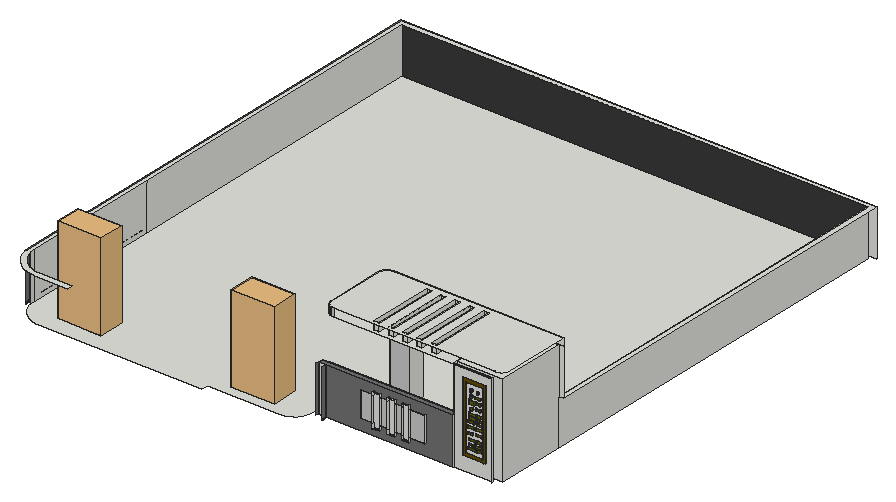
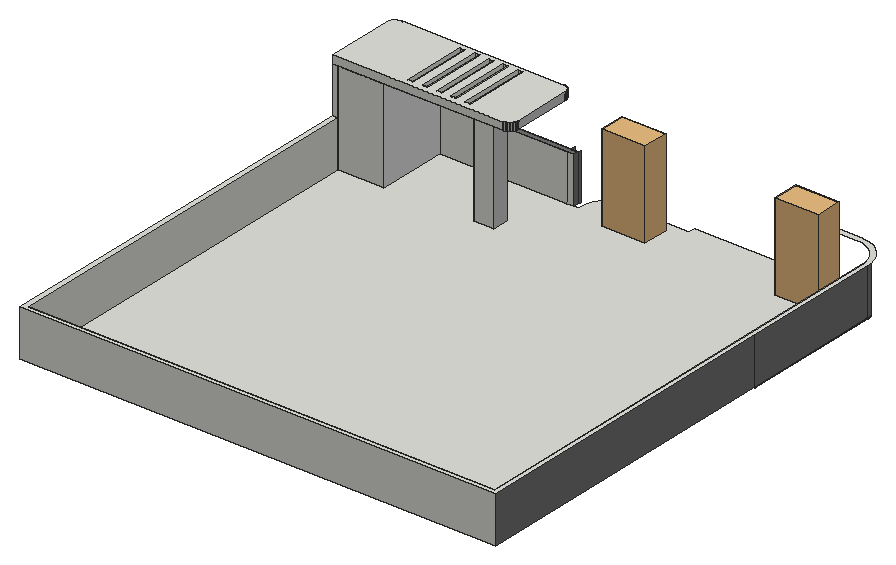
# SketchUp Ruby script. Lengths in inches.
U = 1.inch
M = Sketchup.active_model
def pt(a) = Geom::Point3d.new(a.map { |v| v * U })
def face(e, loops, mat)
  f = e.add_face(loops[0].map { |a| pt(a) })
  loops[1..].each { |l| e.add_face(l.map { |a| pt(a) }).erase! }
  f.material = f.back_material = mat if mat
  f
end
# faces: each face lists its corners as indices into pts; further lists are holes
def faces(e, pts, list, mat = nil) = list.each { |f| face(e, (f[0].is_a?(Array) ? f : [f]).map { |l| l.map { |i| pts[i] } }, mat) }
# xy, xz, yz: faces in a plane at the given z, y or x. An outline is a flat list of corners, or four numbers for a rectangle; further outlines are holes
def ring(l) = l.size == 4 ? [[l[0], l[1]], [l[2], l[1]], [l[2], l[3]], [l[0], l[3]]] : l.each_slice(2).to_a
def flat(e, list, mat, &to3) = list.each { |f| face(e, (f[0].is_a?(Array) ? f : [f]).map { |l| ring(l).map { |u, v| to3.(u, v) } }, mat) }
def xy(e, z, list, mat = nil) = flat(e, list, mat) { |x, y| [x, y, z] }
def xz(e, y, list, mat = nil) = flat(e, list, mat) { |x, z| [x, y, z] }
def yz(e, x, list, mat = nil) = flat(e, list, mat) { |y, z| [x, y, z] }
def lines(e, pts, list) = list.each { |a, b| e.add_line(pt(pts[a]), pt(pts[b])) }
# prism: a flat outline (further loops are holes) pulled along v
def prism(e, loops, v, mat = nil)
  f = face(e, loops, mat); d = Geom::Vector3d.new(v.map { |x| x * U })
  f.pushpull(f.normal.samedirection?(d) ? d.length : -d.length)
end
def box(e, o, s, mat = nil) = prism(e, [[o, [o[0] + s[0], o[1], o[2]], [o[0] + s[0], o[1] + s[1], o[2]], [o[0], o[1] + s[1], o[2]]]], [0, 0, s[2]], mat)
def at(x, y, z, deg = 0) = Geom::Transformation.translation(pt([x, y, z])) * Geom::Transformation.rotation(ORIGIN, Z_AXIS, deg.degrees)
def axes(o, x, y, z) = Geom::Transformation.new([*x, 0, *y, 0, *z, 0, *pt(o).to_a, 1])
def part(name) = M.definitions.add(name)
# library, detail: a bought-in or finely detailed component or shape, given as its bounding box
def library(name, o, s) = part(name).tap { |d| box(d.entities, o, s) }
def detail(e, o, s) = box(e.add_group.entities, o, s)
def put(e, d, t, mat = nil) = e.add_instance(d, t).tap { |i| i.material = mat if mat }
def group(e, t, mat = nil) = e.add_group.tap { |g| g.transformation = t; g.material = mat if mat }.entities
root = M.entities
M.materials.add("[Cladding Stucco White]").color = [200, 200, 200]
M.materials.add("[Color D08]").color = [102, 76, 0]
M.materials.add("[Color E08]").color = [102, 102, 0]
M.materials.add("[Color M01]").color = [226, 226, 226]
M.materials.add("[Color M05]").color = [114, 114, 114]
M.materials.add("[Color M07]").color = [58, 58, 58]
c1 = library("Plant 260 020",[-18.86,-7.03,0.01],[33.61,20.04,67.26])
xy(root,252,[[[24.37,4.65,150.375,4.65,150.375,10.04,205.76,10.04,207.83,10.17,209.75,10.55,211.6,11.18,213.35,12.05,214.98,13.13,216.45,14.42,217.74,15.9,218.83,17.52,219.69,19.28,220.32,21.13,220.7,23.05,221.07,28.65,328.65,28.65,328.65,82.27,364.23,82.27,364.23,381.35,3.9,381.35,3.9,25.12,4.08,22.34,4.6,19.73,5.45,17.21,6.63,14.83,8.11,12.61,9.86,10.61,11.86,8.86,14.08,7.38,16.46,6.2,18.98,5.35,21.59,4.83],[244.86,68.42,260.42,80.36]],[229.875,24.5625,328.65,25]])
xy(root,257.79,[[267.39,23,273.02,24.5625],[279.08,23,284.71,24.5625],[290.02,23,295.64,24.5625]])
xy(root,261.06,[[257.61,24,267.39,24.5625],[273.02,24,279.08,24.5625],[284.71,24,290.02,24.5625],[295.64,24,307.42,24.5625]])
xy(root,262.61,[[336.12,24.6,353.93,25]])
xy(root,264.9375,[[338.45,24.6,351.61,25]],"[Color D08]")
xy(root,268.33,[[340.3,24.6,345.92,25]])
xy(root,268.45,[[347.23,24.6,350.79,25]])
xy(root,269.83,[[340.3,24.6,345.92,25]],"[Color E08]")
xy(root,270.39,[[347.23,24.6,350.79,25]],"[Color E08]")
xy(root,271.27,[[345.53,24.6,351.15,25]])
xy(root,271.58,[[340.9375,24.6,344.6875,25]])
xy(root,272.77,[[345.53,24.6,351.15,25]],"[Color E08]")
xy(root,272.83,[[340.9375,24.6,344.6875,25]],"[Color E08]")
xy(root,274.45,[[347.23,24.6,350.79,25]])
xy(root,274.58,[[340.52,24.6,346.15,25]])
xy(root,276.08,[[340.52,24.6,346.15,25]],"[Color E08]")
xy(root,276.39,[[347.23,24.6,350.79,25]],"[Color E08]")
xy(root,279.15,[[340.1875,24.6,343.9375,25]])
xy(root,279.31,[[346.11,24.6,351.49,25]])
xy(root,280.31,[[257.61,24,267.39,24.5625],[273.02,24,279.08,24.5625],[284.71,24,290.02,24.5625],[295.64,24,307.42,24.5625]])
xy(root,280.4,[[340.1875,24.6,343.9375,25]],"[Color E08]")
xy(root,280.87,[[346.11,24.6,351.49,25]],"[Color E08]")
xy(root,283.04,[[267.39,23,273.02,24.5625],[290.02,23,295.64,24.5625]])
xy(root,283.04,[[279.08,23,284.71,24.5625]],"[Color M01]")
xy(root,283.31,[[340.11,24.6,345.49,25],[346.11,24.6,351.49,25]])
xy(root,284.87,[[340.11,24.6,345.49,25],[346.11,24.6,351.49,25]],"[Color E08]")
xy(root,286.82,[[347.26,24.6,351.01,25]])
xy(root,286.87,[[340.11,24.6,345.49,25]])
xy(root,288,[[24.25,1,49.81,1,49.81,4.65,24.37,4.65,21.59,4.83,18.98,5.35,16.46,6.2,14.08,7.38,11.86,8.86,9.86,10.61,8.11,12.61,6.63,14.83,5.45,17.21,4.6,19.73,4.08,22.34,3.9,25.12,3.9,381.35,364.23,381.35,364.23,82.27,367.875,82.27,367.875,385,0.25,385,0.25,25,0.46,21.87,1.07,18.79,2.08,15.82,3.47,13,5.21,10.39,7.28,8.03,9.64,5.96,12.25,4.22,15.07,2.83,18.04,1.82,21.12,1.21]])
xy(root,288,[[229.875,24.5625,328.65,24.5625,328.65,28.65,224.48,28.65,224.48,25,229.875,25]],"[Color M05]")
xy(root,288.07,[[347.26,24.6,351.01,25]],"[Color E08]")
xy(root,288.43,[[340.11,24.6,345.49,25]],"[Color E08]")
xy(root,289.68,[[340.68,24.6,346.49,25]])
xy(root,289.75,[[347.26,24.6,351.01,25]])
xy(root,291,[[347.26,24.6,351.01,25]],"[Color E08]")
xy(root,291.43,[[340.68,24.6,346.49,25]],"[Color E08]")
xy(root,292.39,[[340.52,24.6,346.15,25]])
xy(root,292.44,[[346.69,24.6,350.25,25]])
xy(root,293.89,[[340.52,24.6,346.15,25]],"[Color E08]")
xy(root,294.38,[[346.69,24.6,350.25,25]],"[Color E08]")
xy(root,296.78,[[346.22,24.6,350.21,25]])
xy(root,298.625,[[346.22,24.6,350.21,25]],"[Color E08]")
xy(root,300.12,[[340.54,24.6,344.89,25]])
xy(root,300.97,[[345.92,24.6,349.92,25]])
xy(root,302.59,[[345.92,24.6,349.92,25]],"[Color E08]")
xy(root,302.8,[[340.54,24.6,344.89,25]],"[Color E08]")
xy(root,305.05,[[345.58,24.6,350.08,25]])
xy(root,306.3,[[345.58,24.6,350.08,25]],"[Color E08]")
xy(root,314.59,[[338.45,24.6,351.61,25]])
xy(root,316.92,[[336.12,24.6,353.93,25]],"[Color D08]")
xy(root,324,[[[236.52,24,235.66,24.06,234.8,24.23,233.98,24.51,233.2,24.89,232.48,25.375,231.82,25.95,231.25,26.6,230.77,27.32,230.38,28.1,230.1,28.93,229.93,29.78,229.875,30.65,229.875,75.46,229.93,76.35,230.11,77.22,230.39,78.07,230.79,78.86,231.28,79.61,231.87,80.28,232.54,80.86,233.28,81.36,234.08,81.75,234.92,82.04,235.8,82.21,236.6875,82.27,328.65,82.27,328.65,25,358.875,25,358.875,24],[265.73,27.1,269.54,77.6],[276.79,27.1,280.6,77.6],[287.85,27.1,291.66,77.6],[298.91,27.1,302.73,77.6],[309.98,27.1,313.79,77.6],[244.86,68.42,260.42,80.36]],[328.65,28.65,364.23,82.27]])
xy(root,330,[[361.5,23.99,361.5625,24,360.74,24],[[236.52,24,361.5625,24,362.25,24.07,362.99,24.22,363.72,24.45,364.41,24.76,365.07,25.14,365.68,25.58,366.24,26.09,366.75,26.65,367.19,27.27,367.57,27.92,367.875,28.62,367.875,82.27,236.6875,82.27,235.8,82.21,234.92,82.04,234.08,81.75,233.28,81.36,232.54,80.86,231.87,80.28,231.28,79.61,230.79,78.86,230.39,78.07,230.11,77.22,229.93,76.35,229.875,75.46,229.875,30.65,229.93,29.78,230.1,28.93,230.38,28.1,230.77,27.32,231.25,26.6,231.82,25.95,232.48,25.375,233.2,24.89,233.98,24.51,234.8,24.23,235.66,24.06],[265.73,27.1,269.54,77.6],[276.79,27.1,280.6,77.6],[287.85,27.1,291.66,77.6],[309.98,27.1,313.79,77.6],[298.91,27.1,302.73,77.6]]])
xz(root,24,[[257.61,261.06,267.39,280.31],[273.02,261.06,279.08,280.31],[284.71,261.06,290.02,280.31],[295.64,261.06,307.42,280.31]],"[Cladding Stucco White]")
xz(root,24.5625,[[[229.875,252,328.65,288],[267.39,257.79,267.39,261.06,257.61,261.06,257.61,280.31,267.39,280.31,267.39,283.04,273.02,283.04,273.02,280.31,279.08,280.31,279.08,283.04,284.71,283.04,284.71,280.31,290.02,280.31,290.02,283.04,295.64,283.04,295.64,280.31,307.42,280.31,307.42,261.06,295.64,261.06,295.64,257.79,290.02,257.79,290.02,261.06,284.71,261.06,284.71,257.79,279.08,257.79,279.08,261.06,273.02,261.06,273.02,257.79]]],"[Color M05]")
xz(root,24.6,[[[336.12,262.61,353.93,316.92],[338.45,264.9375,351.61,314.59]]],"[Color D08]")
xz(root,24.6,[[340.3,268.33,345.92,269.83],[347.23,268.45,350.79,270.39],[345.53,271.27,351.15,272.77],[340.9375,271.58,344.6875,272.83],[347.23,274.45,350.79,276.39],
  [340.52,274.58,346.15,276.08],[340.1875,279.15,343.9375,280.4],[346.11,279.31,351.49,280.87],[340.11,283.31,345.49,284.87],[346.11,283.31,351.49,284.87],
  [347.26,286.82,351.01,288.07],[340.11,286.87,345.49,288.43],[340.68,289.68,346.49,291.43],[347.26,289.75,351.01,291],[340.52,292.39,346.15,293.89],
  [346.69,292.44,350.25,294.38],[343.01,295.6,343.3125,295.64,343.6,295.76,343.85,295.94,344.03,296.19,344.15,296.48,344.19,296.78,344.15,297.09,344.03,297.38,343.85,297.625,343.6,297.8125,343.3125,297.93,343.01,297.97,342.7,297.93,342.41,297.8125,342.17,297.625,341.98,297.38,341.86,297.09,341.82,296.78,341.86,296.48,341.98,296.19,342.17,295.94,342.41,295.76,342.7,295.64],[346.22,296.78,350.21,298.625],[340.54,300.12,344.89,302.8],[345.92,300.97,349.92,302.59],
  [342.68,304.3125,342.98,304.35,343.25,304.46,343.48,304.64,343.66,304.875,343.77,305.15,343.81,305.4375,343.77,305.73,343.66,306,343.48,306.23,343.25,306.41,342.98,306.52,342.68,306.5625,342.39,306.52,342.12,306.41,341.89,306.23,341.71,306,341.6,305.73,341.56,305.4375,341.6,305.15,341.71,304.875,341.89,304.64,342.12,304.46,342.39,304.35],[345.58,305.05,350.08,306.3],[342.68,308.51,342.99,308.55,343.28,308.67,343.52,308.86,343.71,309.11,343.83,309.39,343.87,309.7,343.83,310.01,343.71,310.3,343.52,310.54,343.28,310.73,342.99,310.85,342.68,310.89,342.375,310.85,342.09,310.73,341.84,310.54,341.66,310.3,341.54,310.01,341.5,309.7,341.54,309.39,341.66,309.11,341.84,308.86,342.09,308.67,342.375,308.55],[347.69,308.5625,347.93,308.6,348.16,308.6875,348.35,308.84,348.5,309.03,348.6,309.26,348.63,309.5,348.6,309.74,348.5,309.97,348.35,310.16,348.16,310.3125,347.93,310.41,347.69,310.4375,347.45,310.41,347.22,310.3125,347.03,310.16,346.88,309.97,346.79,309.74,346.75,309.5,346.79,309.26,346.88,309.03,347.03,308.84,347.22,308.6875,347.45,308.6]],"[Color E08]")
xz(root,25,[[224.48,252,229.875,288],[[328.65,252,358.875,324],[336.12,262.61,353.93,316.92]]])
xz(root,25,[[[338.45,264.9375,351.61,314.59],[340.54,300.12,344.89,302.8],[340.68,289.68,346.49,291.43],[340.52,292.39,346.15,293.89],[340.52,274.58,346.15,276.08],[345.53,271.27,351.15,272.77],[340.3,268.33,345.92,269.83],[340.11,286.87,345.49,288.43],[340.11,283.31,345.49,284.87],[346.11,283.31,351.49,284.87],[346.11,279.31,351.49,280.87],[346.22,296.78,350.21,298.625],[346.69,292.44,350.25,294.38],[347.23,274.45,350.79,276.39],[347.23,268.45,350.79,270.39],[345.92,300.97,349.92,302.59],[345.58,305.05,350.08,306.3],[347.26,289.75,351.01,291],[347.26,286.82,351.01,288.07],[340.1875,279.15,343.9375,280.4],[340.9375,271.58,344.6875,272.83],[342.68,308.51,342.375,308.55,342.09,308.67,341.84,308.86,341.66,309.11,341.54,309.39,341.5,309.7,341.54,310.01,341.66,310.3,341.84,310.54,342.09,310.73,342.375,310.85,342.68,310.89,342.99,310.85,343.28,310.73,343.52,310.54,343.71,310.3,343.83,310.01,343.87,309.7,343.83,309.39,343.71,309.11,343.52,308.86,343.28,308.67,342.99,308.55],[343.01,295.6,342.7,295.64,342.41,295.76,342.17,295.94,341.98,296.19,341.86,296.48,341.82,296.78,341.86,297.09,341.98,297.38,342.17,297.625,342.41,297.8125,342.7,297.93,343.01,297.97,343.3125,297.93,343.6,297.8125,343.85,297.625,344.03,297.38,344.15,297.09,344.19,296.78,344.15,296.48,344.03,296.19,343.85,295.94,343.6,295.76,343.3125,295.64],[342.68,304.3125,342.39,304.35,342.12,304.46,341.89,304.64,341.71,304.875,341.6,305.15,341.56,305.4375,341.6,305.73,341.71,306,341.89,306.23,342.12,306.41,342.39,306.52,342.68,306.5625,342.98,306.52,343.25,306.41,343.48,306.23,343.66,306,343.77,305.73,343.81,305.4375,343.77,305.15,343.66,304.875,343.48,304.64,343.25,304.46,342.98,304.35],[347.69,308.5625,347.45,308.6,347.22,308.6875,347.03,308.84,346.88,309.03,346.79,309.26,346.75,309.5,346.79,309.74,346.88,309.97,347.03,310.16,347.22,310.3125,347.45,310.41,347.69,310.4375,347.93,310.41,348.16,310.3125,348.35,310.16,348.5,309.97,348.6,309.74,348.63,309.5,348.6,309.26,348.5,309.03,348.35,308.84,348.16,308.6875,347.93,308.6]]],"[Color M01]")
xz(root,27.1,[[265.73,324,269.54,330],[276.79,324,280.6,330],[287.85,324,291.66,330],[298.91,324,302.73,330],[309.98,324,313.79,330]])
xz(root,28.65,[[224.48,252,229.875,288],[229.875,252,328.65,288],[328.65,252,364.23,324]])
xz(root,68.42,[[244.86,252,260.42,324]],"[Cladding Stucco White]")
xz(root,77.6,[[265.73,324,269.54,330],[276.79,324,280.6,330],[287.85,324,291.66,330],[298.91,324,302.73,330],[309.98,324,313.79,330]])
xz(root,80.36,[[244.86,252,260.42,324]])
xz(root,82.27,[[328.65,252,364.23,324],[364.23,288,367.875,324],[236.6875,324,367.875,330]])
xz(root,134.58,[[0.25,251.0625,0.18,251.12,0.12,251.1875,0.07,251.27,0.03,251.35,0.01,251.4375,0,251.53,0.01,251.625,0.03,251.71,0.07,251.8,0.12,251.875,0.18,251.94,0.25,252]])
xz(root,381.35,[[3.9,252,364.23,288]],"[Color M07]")
xz(root,385,[[0.25,252,367.875,288]])
yz(root,0.25,[[25,252,134.58,288],[134.58,252,385,288]],"[Color M05]")
yz(root,3.9,[[25.12,252,134.58,288],[134.58,252,381.35,288]])
yz(root,224.48,[[25,252,28.65,288]],"[Color M05]")
yz(root,229.875,[[24.5625,252,25,288]])
yz(root,229.875,[[30.65,324,75.46,330]],"[Cladding Stucco White]")
yz(root,244.86,[[68.42,252,80.36,324]],"[Cladding Stucco White]")
yz(root,257.61,[[24,261.06,24.5625,280.31]])
yz(root,260.42,[[68.42,252,80.36,324]])
yz(root,265.73,[[27.1,324,77.6,330]])
yz(root,267.39,[[23,257.79,24.5625,261.06],[23,261.06,24,280.31],[23,280.31,24.5625,283.04]])
yz(root,269.54,[[27.1,324,77.6,330]])
yz(root,273.02,[[23,257.79,24.5625,261.06]])
yz(root,273.02,[[23,261.06,24,280.31],[23,280.31,24.5625,283.04]],"[Color M01]")
yz(root,276.79,[[27.1,324,77.6,330]])
yz(root,279.08,[[23,257.79,24.5625,261.06],[23,261.06,24,280.31],[23,280.31,24.5625,283.04]])
yz(root,280.6,[[27.1,324,77.6,330]])
yz(root,284.71,[[23,257.79,24.5625,261.06],[23,261.06,24,280.31]])
yz(root,284.71,[[23,280.31,24.5625,283.04]],"[Color M01]")
yz(root,287.85,[[27.1,324,77.6,330]])
yz(root,290.02,[[23,257.79,24.5625,261.06],[23,261.06,24,280.31],[23,280.31,24.5625,283.04]])
yz(root,291.66,[[27.1,324,77.6,330]])
yz(root,295.64,[[23,257.79,24.5625,261.06],[23,261.06,24,280.31],[23,280.31,24.5625,283.04]])
yz(root,298.91,[[27.1,324,77.6,330]])
yz(root,302.73,[[27.1,324,77.6,330]])
yz(root,307.42,[[24,261.06,24.5625,280.31]])
yz(root,309.98,[[27.1,324,77.6,330]])
yz(root,313.79,[[27.1,324,77.6,330]])
yz(root,328.65,[[24.5625,252,25,288],[25,288,28.65,324]])
yz(root,328.65,[[28.65,252,82.27,324]],"[Color M01]")
yz(root,336.12,[[24.6,262.61,25,316.92]],"[Color D08]")
yz(root,338.45,[[24.6,264.9375,25,314.59]],"[Color D08]")
yz(root,340.11,[[24.6,283.31,25,284.87],[24.6,286.87,25,288.43]],"[Color E08]")
yz(root,340.1875,[[24.6,279.15,25,280.4]],"[Color E08]")
yz(root,340.3,[[24.6,268.33,25,269.83]],"[Color E08]")
yz(root,340.52,[[24.6,274.58,25,276.08],[24.6,292.39,25,293.89]],"[Color E08]")
yz(root,340.54,[[24.6,300.12,25,302.8]],"[Color E08]")
yz(root,340.68,[[24.6,289.68,25,291.43]],"[Color E08]")
yz(root,340.9375,[[24.6,271.58,25,272.83]],"[Color E08]")
yz(root,343.9375,[[24.6,279.15,25,280.4]],"[Color E08]")
yz(root,344.6875,[[24.6,271.58,25,272.83]],"[Color E08]")
yz(root,344.89,[[24.6,300.12,25,302.8]],"[Color E08]")
yz(root,345.49,[[24.6,283.31,25,284.87],[24.6,286.87,25,288.43]],"[Color E08]")
yz(root,345.53,[[24.6,271.27,25,272.77]],"[Color E08]")
yz(root,345.58,[[24.6,305.05,25,306.3]],"[Color E08]")
yz(root,345.92,[[24.6,268.33,25,269.83],[24.6,300.97,25,302.59]],"[Color E08]")
yz(root,346.11,[[24.6,279.31,25,280.87],[24.6,283.31,25,284.87]],"[Color E08]")
yz(root,346.15,[[24.6,274.58,25,276.08],[24.6,292.39,25,293.89]],"[Color E08]")
yz(root,346.22,[[24.6,296.78,25,298.625]],"[Color E08]")
yz(root,346.49,[[24.6,289.68,25,291.43]],"[Color E08]")
yz(root,346.69,[[24.6,292.44,25,294.38]],"[Color E08]")
yz(root,347.23,[[24.6,268.45,25,270.39],[24.6,274.45,25,276.39]],"[Color E08]")
yz(root,347.26,[[24.6,286.82,25,288.07],[24.6,289.75,25,291]],"[Color E08]")
yz(root,349.92,[[24.6,300.97,25,302.59]],"[Color E08]")
yz(root,350.08,[[24.6,305.05,25,306.3]],"[Color E08]")
yz(root,350.21,[[24.6,296.78,25,298.625]],"[Color E08]")
yz(root,350.25,[[24.6,292.44,25,294.38]],"[Color E08]")
yz(root,350.79,[[24.6,268.45,25,270.39],[24.6,274.45,25,276.39]],"[Color E08]")
yz(root,351.01,[[24.6,286.82,25,288.07],[24.6,289.75,25,291]],"[Color E08]")
yz(root,351.15,[[24.6,271.27,25,272.77]],"[Color E08]")
yz(root,351.49,[[24.6,279.31,25,280.87],[24.6,283.31,25,284.87]],"[Color E08]")
yz(root,351.61,[[24.6,264.9375,25,314.59]],"[Color D08]")
yz(root,353.93,[[24.6,262.61,25,316.92]],"[Color D08]")
yz(root,358.875,[[24,252,25,324]])
yz(root,364.23,[[28.65,252,82.27,324],[82.27,252,381.35,288]])
p = [[0.12,25,251.1875],[0.18,25,251.12],[0.38,21.86,251.12],[0.32,21.85,251.1875],[229.8,21.85,251.1875],[229.74,21.86,251.12],
  [229.95,25,251.12],[230.01,24.99,251.1875],[0.25,25,251.0625],[0.46,21.87,251.0625],[229.67,21.87,251.0625],[229.875,25,251.0625],
  [0.12,134.58,251.1875],[0.18,134.58,251.12],[0.25,134.58,251.0625],[229.875,25,252],[229.95,25,251.94],[230.01,24.99,251.875],
  [230.06,24.99,251.8],[230.09,24.99,251.71],[230.12,24.98,251.625],[230.125,24.98,251.53],[230.12,24.98,251.4375],[230.09,24.99,251.35],
  [230.06,24.99,251.27],[0.07,24.99,251.27],[0.27,21.84,251.27],[229.85,21.84,251.27],[0.07,134.58,251.27],[0.03,24.99,251.35],
  [0.24,21.84,251.35],[229.89,21.84,251.35],[0.03,134.58,251.35],[0,24.99,251.53],[0.01,24.99,251.4375],[0.21,21.84,251.4375],
  [0.21,21.83,251.53],[229.91,21.84,251.4375],[0,134.58,251.53],[0.01,134.58,251.4375],[0.01,24.99,251.625],[0.21,21.84,251.625],
  [0.01,134.58,251.625],[0.03,24.99,251.71],[0.24,21.84,251.71],[229.89,21.84,251.71],[229.91,21.84,251.625],[0.03,134.58,251.71],
  [0.07,24.99,251.8],[0.27,21.84,251.8],[229.85,21.84,251.8],[0.07,134.58,251.8],[0.12,25,251.875],[0.32,21.85,251.875],
  [229.8,21.85,251.875],[0.12,134.58,251.875],[0.18,25,251.94],[0.38,21.86,251.94],[229.74,21.86,251.94],[0.25,25,252],
  [0.46,21.87,252],[229.67,21.87,252],[0.18,134.58,251.94],[0.25,134.58,252],[0.46,21.87,288],[0.25,25,288],
  [229.875,25,288],[229.67,21.87,288],[4.08,22.34,252],[3.9,25.12,252],[3.9,25.12,288],[4.08,22.34,288],
  [224.48,25,252],[224.32,22.57,252],[224.32,22.57,288],[224.48,25,288],[342.41,25,295.76],[342.7,25,295.64],
  [342.7,24.6,295.64],[342.41,24.6,295.76],[343.01,25,295.6],[343.01,24.6,295.6],[343.3125,25,295.64],[343.3125,24.6,295.64],
  [343.6,25,295.76],[343.6,24.6,295.76],[342.17,25,295.94],[342.17,24.6,295.94],[343.85,25,295.94],[343.85,24.6,295.94],
  [341.98,25,296.19],[341.98,24.6,296.19],[344.03,25,296.19],[344.03,24.6,296.19],[341.86,25,296.48],[341.86,24.6,296.48],
  [344.15,25,296.48],[344.15,24.6,296.48],[341.82,25,296.78],[341.82,24.6,296.78],[344.19,25,296.78],[344.19,24.6,296.78],
  [341.86,25,297.09],[341.86,24.6,297.09],[344.15,25,297.09],[344.15,24.6,297.09],[341.98,25,297.38],[341.98,24.6,297.38],
  [344.03,25,297.38],[344.03,24.6,297.38],[342.17,25,297.625],[342.17,24.6,297.625],[343.85,25,297.625],[343.85,24.6,297.625],
  [342.41,25,297.8125],[342.41,24.6,297.8125],[343.6,25,297.8125],[343.6,24.6,297.8125],[342.7,25,297.93],[342.7,24.6,297.93],
  [343.3125,25,297.93],[343.3125,24.6,297.93],[343.01,25,297.97],[343.01,24.6,297.97],[342.39,25,304.35],[342.68,25,304.3125],
  [342.68,24.6,304.3125],[342.39,24.6,304.35],[342.98,25,304.35],[342.98,24.6,304.35],[342.12,25,304.46],[342.12,24.6,304.46],
  [343.25,25,304.46],[343.25,24.6,304.46],[341.89,25,304.64],[341.89,24.6,304.64],[343.48,25,304.64],[343.48,24.6,304.64],
  [341.71,25,304.875],[341.71,24.6,304.875],[343.66,25,304.875],[343.66,24.6,304.875],[341.6,25,305.15],[341.6,24.6,305.15],
  [343.77,25,305.15],[343.77,24.6,305.15],[341.56,25,305.4375],[341.56,24.6,305.4375],[343.81,25,305.4375],[343.81,24.6,305.4375],
  [341.6,25,305.73],[341.6,24.6,305.73],[343.77,25,305.73],[343.77,24.6,305.73],[341.71,25,306],[341.71,24.6,306],
  [343.66,25,306],[343.66,24.6,306],[341.89,25,306.23],[341.89,24.6,306.23],[343.48,25,306.23],[343.48,24.6,306.23],
  [342.12,25,306.41],[342.12,24.6,306.41],[343.25,25,306.41],[343.25,24.6,306.41],[342.39,25,306.52],[342.39,24.6,306.52],
  [342.98,25,306.52],[342.98,24.6,306.52],[342.68,25,306.5625],[342.68,24.6,306.5625],[342.375,25,308.55],[342.68,25,308.51],
  [342.68,24.6,308.51],[342.375,24.6,308.55],[342.99,25,308.55],[342.99,24.6,308.55],[342.09,25,308.67],[342.09,24.6,308.67],
  [343.28,25,308.67],[343.28,24.6,308.67],[347.22,25,308.6875],[347.45,25,308.6],[347.45,24.6,308.6],[347.22,24.6,308.6875],
  [347.69,25,308.5625],[347.69,24.6,308.5625],[347.93,25,308.6],[347.93,24.6,308.6],[348.16,25,308.6875],[348.16,24.6,308.6875],
  [341.84,25,308.86],[341.84,24.6,308.86],[343.52,25,308.86],[343.52,24.6,308.86],[347.03,25,308.84],[347.03,24.6,308.84],
  [348.35,25,308.84],[348.35,24.6,308.84],[346.88,25,309.03],[346.88,24.6,309.03],[348.5,25,309.03],[348.5,24.6,309.03],
  [341.66,25,309.11],[341.66,24.6,309.11],[343.71,25,309.11],[343.71,24.6,309.11],[346.79,25,309.26],[346.79,24.6,309.26],
  [348.6,25,309.26],[348.6,24.6,309.26],[341.54,25,309.39],[341.54,24.6,309.39],[343.83,25,309.39],[343.83,24.6,309.39],
  [346.75,25,309.5],[346.75,24.6,309.5],[348.63,25,309.5],[348.63,24.6,309.5],[341.5,25,309.7],[341.5,24.6,309.7],
  [343.87,25,309.7],[343.87,24.6,309.7],[346.79,25,309.74],[346.79,24.6,309.74],[348.6,25,309.74],[348.6,24.6,309.74],
  [341.54,25,310.01],[341.54,24.6,310.01],[343.83,25,310.01],[343.83,24.6,310.01],[346.88,25,309.97],[346.88,24.6,309.97],
  [348.5,25,309.97],[348.5,24.6,309.97],[341.66,25,310.3],[341.66,24.6,310.3],[343.71,25,310.3],[343.71,24.6,310.3],
  [347.03,25,310.16],[347.03,24.6,310.16],[348.35,25,310.16],[348.35,24.6,310.16],[347.22,25,310.3125],[347.22,24.6,310.3125],
  [348.16,25,310.3125],[348.16,24.6,310.3125],[341.84,25,310.54],[341.84,24.6,310.54],[343.52,25,310.54],[343.52,24.6,310.54],
  [347.45,25,310.41],[347.45,24.6,310.41],[347.93,25,310.41],[347.93,24.6,310.41],[347.69,25,310.4375],[347.69,24.6,310.4375],
  [342.09,25,310.73],[342.09,24.6,310.73],[343.28,25,310.73],[343.28,24.6,310.73],[342.375,25,310.85],[342.375,24.6,310.85],
  [342.99,25,310.85],[342.99,24.6,310.85],[342.68,25,310.89],[342.68,24.6,310.89],[236.52,24,330],[235.66,24.06,330],
  [235.66,24.06,324],[236.52,24,324],[234.8,24.23,330],[234.8,24.23,324],[233.98,24.51,330],[233.98,24.51,324],
  [233.2,24.89,330],[233.2,24.89,324],[232.48,25.375,330],[232.48,25.375,324],[231.82,25.95,330],[231.82,25.95,324],
  [231.25,26.6,330],[231.25,26.6,324],[230.77,27.32,330],[230.77,27.32,324],[230.38,28.1,330],[230.38,28.1,324],
  [230.1,28.93,330],[230.1,28.93,324],[229.93,29.78,330],[229.93,29.78,324],[229.875,30.65,330],[229.875,30.65,324],
  [229.875,75.46,330],[229.93,76.35,330],[229.93,76.35,324],[229.875,75.46,324],[230.11,77.22,330],[230.11,77.22,324],
  [230.39,78.07,330],[230.39,78.07,324],[230.79,78.86,330],[230.79,78.86,324],[231.28,79.61,330],[231.28,79.61,324],
  [231.87,80.28,330],[231.87,80.28,324],[232.54,80.86,330],[232.54,80.86,324],[233.28,81.36,330],[233.28,81.36,324],
  [234.08,81.75,330],[234.08,81.75,324],[234.92,82.04,330],[234.92,82.04,324],[235.8,82.21,330],[235.8,82.21,324],
  [236.6875,82.27,330],[236.6875,82.27,324],[224.1875,22.68,251.4]]
faces(root,p,[[0,1,2,3],[4,5,6,7],[1,8,9,2],[5,10,11,6],[12,13,1,0],[13,14,8,1],[25,0,3,26],[27,4,7,24],
  [28,12,0,25],[29,25,26,30],[31,27,24,23],[32,28,25,29],[33,34,35,36],[34,29,30,35],[37,31,23,22],[38,39,34,33],
  [39,32,29,34],[40,33,36,41],[42,38,33,40],[43,40,41,44],[45,46,20,19],[47,42,40,43],[48,43,44,49],[50,45,19,18],
  [51,47,43,48],[52,48,49,53],[54,50,18,17],[55,51,48,52],[56,52,53,57],[58,54,17,16],[59,56,57,60],[61,58,16,15],
  [62,55,52,56],[63,62,56,59]],"[Color M07]")
faces(root,p,[[6,11,15,16,17,18,19,20,21,22,23,24,7],[68,69,70,71]])
faces(root,p,[[59,60,64,65],[61,15,66,67],[72,73,74,75]],"[Color M05]")
faces(root,p,[[76,77,78,79],[77,80,81,78],[80,82,83,81],[82,84,85,83],[86,76,79,87],[84,88,89,85],[90,86,87,91],[88,92,93,89],
  [94,90,91,95],[92,96,97,93],[98,94,95,99],[96,100,101,97],[102,98,99,103],[100,104,105,101],[106,102,103,107],[104,108,109,105],
  [110,106,107,111],[108,112,113,109],[114,110,111,115],[112,116,117,113],[118,114,115,119],[116,120,121,117],[122,118,119,123],[120,122,123,121],
  [124,125,126,127],[125,128,129,126],[130,124,127,131],[128,132,133,129],[134,130,131,135],[132,136,137,133],[138,134,135,139],[136,140,141,137],
  [142,138,139,143],[140,144,145,141],[146,142,143,147],[144,148,149,145],[150,146,147,151],[148,152,153,149],[154,150,151,155],[152,156,157,153],
  [158,154,155,159],[156,160,161,157],[162,158,159,163],[160,164,165,161],[166,162,163,167],[164,168,169,165],[170,166,167,171],[168,170,171,169],
  [172,173,174,175],[173,176,177,174],[178,172,175,179],[176,180,181,177],[182,183,184,185],[183,186,187,184],[186,188,189,187],[188,190,191,189],
  [192,178,179,193],[180,194,195,181],[196,182,185,197],[190,198,199,191],[200,196,197,201],[198,202,203,199],[204,192,193,205],[194,206,207,195],
  [208,200,201,209],[202,210,211,203],[212,204,205,213],[206,214,215,207],[216,208,209,217],[210,218,219,211],[220,212,213,221],[214,222,223,215],
  [224,216,217,225],[218,226,227,219],[228,220,221,229],[222,230,231,223],[232,224,225,233],[226,234,235,227],[236,228,229,237],[230,238,239,231],
  [240,232,233,241],[234,242,243,235],[244,240,241,245],[242,246,247,243],[248,236,237,249],[238,250,251,239],[252,244,245,253],[246,254,255,247],
  [256,252,253,257],[254,256,257,255],[258,248,249,259],[250,260,261,251],[262,258,259,263],[260,264,265,261],[266,262,263,267],[264,266,267,265]],"[Color E08]")
faces(root,p,[[268,269,270,271],[269,272,273,270],[272,274,275,273],[274,276,277,275],[276,278,279,277],[278,280,281,279],[280,282,283,281],[282,284,285,283],
  [284,286,287,285],[286,288,289,287],[288,290,291,289],[290,292,293,291],[294,295,296,297],[295,298,299,296],[298,300,301,299],[300,302,303,301],
  [302,304,305,303],[304,306,307,305],[306,308,309,307],[308,310,311,309],[310,312,313,311],[312,314,315,313],[314,316,317,315],[316,318,319,317]],"[Cladding Stucco White]")
lines(root,p,[[320,72]])
put(root,c1,at(181.34,24.7,252))
put(root,c1,at(46.5625,25.27,252))
